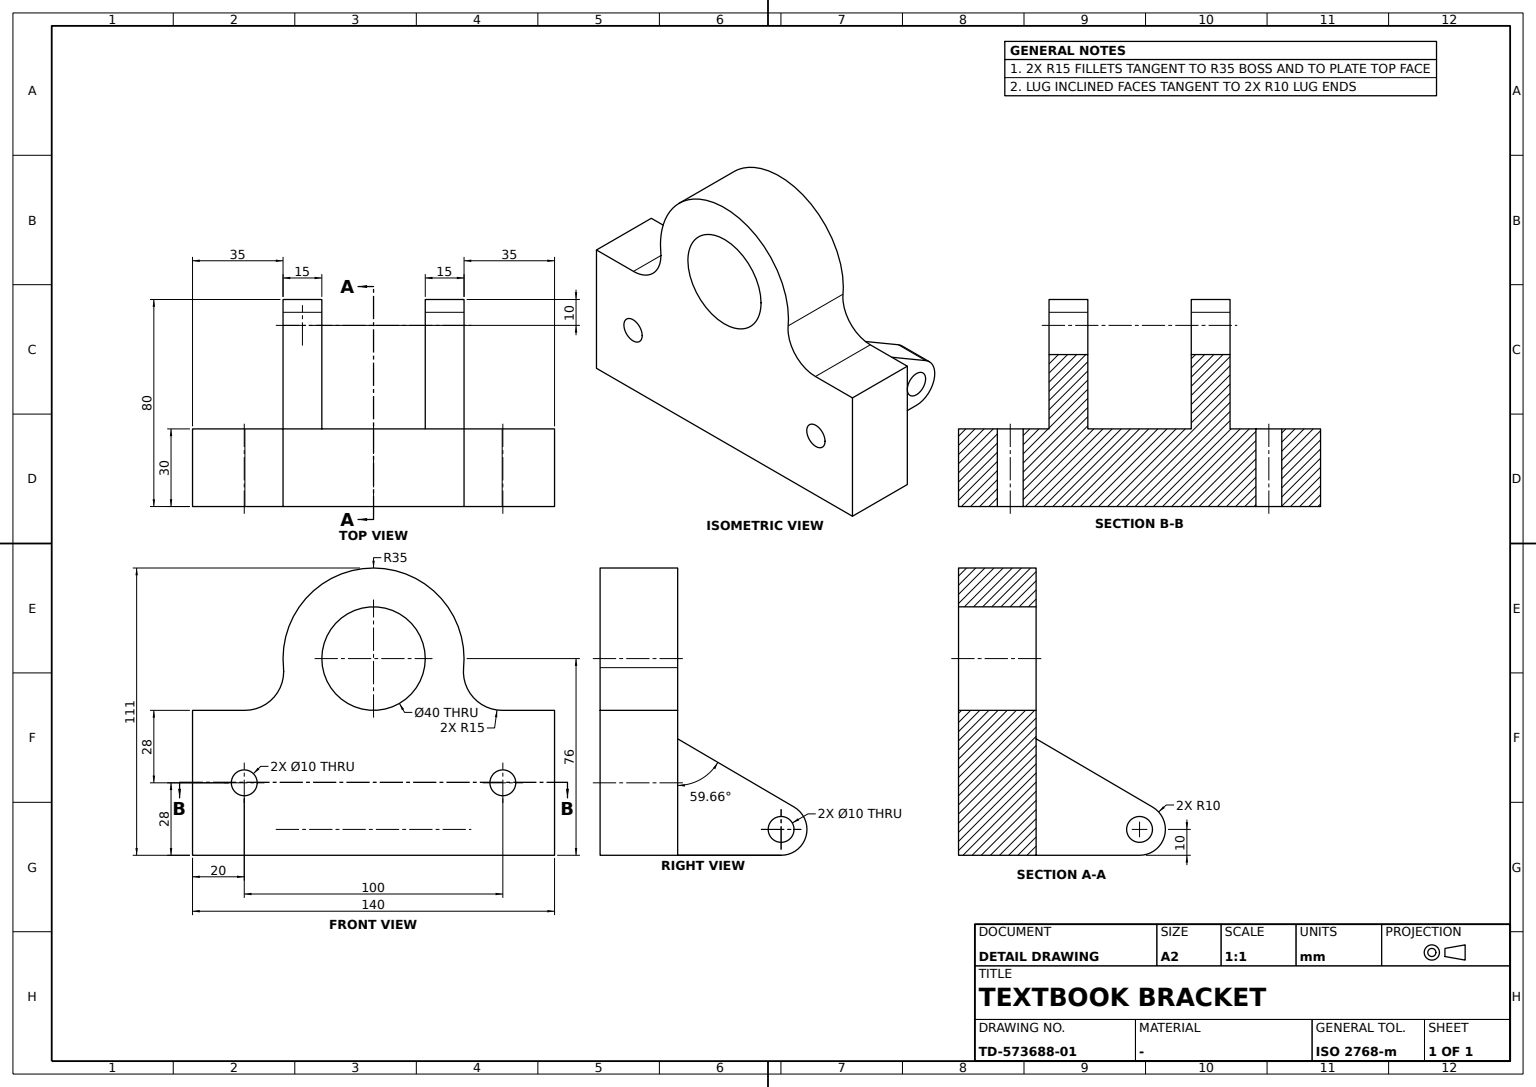
ISO-10303-21;
HEADER;
FILE_DESCRIPTION((''),'2;1');
FILE_NAME('','',(''),(''),'','','');
FILE_SCHEMA(('AUTOMOTIVE_DESIGN'));
ENDSEC;
DATA;
#1=APPLICATION_CONTEXT('');
#2=PRODUCT_CONTEXT('',#1,'mechanical');
#3=PRODUCT('','','',(#2));
#4=PRODUCT_DEFINITION_FORMATION('','',#3);
#5=PRODUCT_DEFINITION_CONTEXT('',#1,'design');
#6=PRODUCT_DEFINITION('','',#4,#5);
#7=PRODUCT_DEFINITION_SHAPE('','',#6);
#8=(LENGTH_UNIT()NAMED_UNIT(*)SI_UNIT(.MILLI.,.METRE.));
#9=(NAMED_UNIT(*)PLANE_ANGLE_UNIT()SI_UNIT($,.RADIAN.));
#10=(NAMED_UNIT(*)SI_UNIT($,.STERADIAN.)SOLID_ANGLE_UNIT());
#11=UNCERTAINTY_MEASURE_WITH_UNIT(LENGTH_MEASURE(1.E-05),#8,'distance_accuracy_value','');
#12=(GEOMETRIC_REPRESENTATION_CONTEXT(3)GLOBAL_UNCERTAINTY_ASSIGNED_CONTEXT((#11))GLOBAL_UNIT_ASSIGNED_CONTEXT((#8,#9,#10))REPRESENTATION_CONTEXT('',''));
#13=CARTESIAN_POINT('',(-40.,-20.,0.));
#14=VERTEX_POINT('',#13);
#15=CARTESIAN_POINT('',(-50.,-20.,10.));
#16=VERTEX_POINT('',#15);
#17=CARTESIAN_POINT('',(-40.,-20.,10.));
#18=DIRECTION('',(0.,1.,0.));
#19=DIRECTION('',(-1.,0.,0.));
#20=AXIS2_PLACEMENT_3D('',#17,#18,#19);
#21=CIRCLE('',#20,10.);
#22=EDGE_CURVE('',#14,#16,#21,.T.);
#23=ORIENTED_EDGE('',*,*,#22,.T.);
#24=CARTESIAN_POINT('',(-45.051517,-20.,18.630305));
#25=VERTEX_POINT('',#24);
#26=EDGE_CURVE('',#16,#25,#21,.T.);
#27=ORIENTED_EDGE('',*,*,#26,.T.);
#28=CARTESIAN_POINT('',(0.,-20.,45.));
#29=VERTEX_POINT('',#28);
#30=CARTESIAN_POINT('',(-22.525759,-20.,31.815153));
#31=DIRECTION('',(0.863030549,0.,0.505151731));
#32=VECTOR('',#31,1000.);
#33=LINE('',#30,#32);
#34=EDGE_CURVE('',#25,#29,#33,.T.);
#35=ORIENTED_EDGE('',*,*,#34,.T.);
#36=CARTESIAN_POINT('',(0.,-20.,0.));
#37=VERTEX_POINT('',#36);
#38=CARTESIAN_POINT('',(0.,-20.,22.5));
#39=DIRECTION('',(0.,0.,-1.));
#40=VECTOR('',#39,1000.);
#41=LINE('',#38,#40);
#42=EDGE_CURVE('',#29,#37,#41,.T.);
#43=ORIENTED_EDGE('',*,*,#42,.T.);
#44=CARTESIAN_POINT('',(-20.,-20.,0.));
#45=VECTOR('',#19,1000.);
#46=LINE('',#44,#45);
#47=EDGE_CURVE('',#37,#14,#46,.T.);
#48=ORIENTED_EDGE('',*,*,#47,.T.);
#49=EDGE_LOOP('',(#23,#27,#35,#43,#48));
#50=FACE_OUTER_BOUND('',#49,.T.);
#51=CARTESIAN_POINT('',(-35.,-20.,10.));
#52=VERTEX_POINT('',#51);
#53=CARTESIAN_POINT('',(-45.,-20.,10.));
#54=VERTEX_POINT('',#53);
#55=CIRCLE('',#20,5.);
#56=EDGE_CURVE('',#52,#54,#55,.T.);
#57=ORIENTED_EDGE('',*,*,#56,.F.);
#58=EDGE_CURVE('',#54,#52,#55,.T.);
#59=ORIENTED_EDGE('',*,*,#58,.F.);
#60=EDGE_LOOP('',(#57,#59));
#61=FACE_BOUND('',#60,.T.);
#62=AXIS2_PLACEMENT_3D('',#36,#18,#19);
#63=PLANE('',#62);
#64=ADVANCED_FACE('',(#50,#61),#63,.T.);
#65=ORIENTED_EDGE('',*,*,#22,.F.);
#66=CARTESIAN_POINT('',(-40.,-35.,0.));
#67=VERTEX_POINT('',#66);
#68=CARTESIAN_POINT('',(-40.,-27.5,0.));
#69=DIRECTION('',(0.,-1.,0.));
#70=VECTOR('',#69,1000.);
#71=LINE('',#68,#70);
#72=EDGE_CURVE('',#14,#67,#71,.T.);
#73=ORIENTED_EDGE('',*,*,#72,.T.);
#74=CARTESIAN_POINT('',(-50.,-35.,10.));
#75=VERTEX_POINT('',#74);
#76=CARTESIAN_POINT('',(-40.,-35.,10.));
#77=AXIS2_PLACEMENT_3D('',#76,#18,#19);
#78=CIRCLE('',#77,10.);
#79=EDGE_CURVE('',#67,#75,#78,.T.);
#80=ORIENTED_EDGE('',*,*,#79,.T.);
#81=CARTESIAN_POINT('',(-50.,27.5,10.));
#82=LINE('',#81,#70);
#83=EDGE_CURVE('',#16,#75,#82,.T.);
#84=ORIENTED_EDGE('',*,*,#83,.F.);
#85=EDGE_LOOP('',(#65,#73,#80,#84));
#86=FACE_OUTER_BOUND('',#85,.T.);
#87=CARTESIAN_POINT('',(-40.,27.5,10.));
#88=AXIS2_PLACEMENT_3D('',#87,#69,#19);
#89=CYLINDRICAL_SURFACE('',#88,10.);
#90=ADVANCED_FACE('',(#86),#89,.T.);
#91=CARTESIAN_POINT('',(0.,-34.82456,72.5));
#92=VERTEX_POINT('',#91);
#93=CARTESIAN_POINT('',(30.,-34.82456,72.5));
#94=VERTEX_POINT('',#93);
#95=CARTESIAN_POINT('',(15.,-34.82456,72.5));
#96=DIRECTION('',(1.,0.,0.));
#97=VECTOR('',#96,1000.);
#98=LINE('',#95,#97);
#99=EDGE_CURVE('',#92,#94,#98,.T.);
#100=ORIENTED_EDGE('',*,*,#99,.F.);
#101=CARTESIAN_POINT('',(0.,-34.749372,71.));
#102=VERTEX_POINT('',#101);
#103=CARTESIAN_POINT('',(0.,-49.749372,71.));
#104=AXIS2_PLACEMENT_3D('',#103,#19,#18);
#105=CIRCLE('',#104,15.);
#106=EDGE_CURVE('',#92,#102,#105,.T.);
#107=ORIENTED_EDGE('',*,*,#106,.T.);
#108=CARTESIAN_POINT('',(30.,-34.749372,71.));
#109=VERTEX_POINT('',#108);
#110=CARTESIAN_POINT('',(15.,-34.749372,71.));
#111=LINE('',#110,#45);
#112=EDGE_CURVE('',#109,#102,#111,.T.);
#113=ORIENTED_EDGE('',*,*,#112,.F.);
#114=CARTESIAN_POINT('',(30.,-49.749372,71.));
#115=AXIS2_PLACEMENT_3D('',#114,#19,#18);
#116=CIRCLE('',#115,15.);
#117=EDGE_CURVE('',#94,#109,#116,.T.);
#118=ORIENTED_EDGE('',*,*,#117,.F.);
#119=EDGE_LOOP('',(#100,#107,#113,#118));
#120=FACE_OUTER_BOUND('',#119,.T.);
#121=CARTESIAN_POINT('',(15.,-49.749372,71.));
#122=AXIS2_PLACEMENT_3D('',#121,#19,#18);
#123=CYLINDRICAL_SURFACE('',#122,15.);
#124=ADVANCED_FACE('',(#120),#123,.F.);
#125=CARTESIAN_POINT('',(30.,35.,76.));
#126=VERTEX_POINT('',#125);
#127=CARTESIAN_POINT('',(0.,35.,76.));
#128=VERTEX_POINT('',#127);
#129=CARTESIAN_POINT('',(15.,35.,76.));
#130=LINE('',#129,#45);
#131=EDGE_CURVE('',#126,#128,#130,.T.);
#132=ORIENTED_EDGE('',*,*,#131,.T.);
#133=CARTESIAN_POINT('',(0.,-35.,76.));
#134=VERTEX_POINT('',#133);
#135=CARTESIAN_POINT('',(0.,0.,76.));
#136=AXIS2_PLACEMENT_3D('',#135,#96,#18);
#137=CIRCLE('',#136,35.);
#138=EDGE_CURVE('',#128,#134,#137,.T.);
#139=ORIENTED_EDGE('',*,*,#138,.T.);
#140=CARTESIAN_POINT('',(30.,-35.,76.));
#141=VERTEX_POINT('',#140);
#142=CARTESIAN_POINT('',(15.,-35.,76.));
#143=LINE('',#142,#45);
#144=EDGE_CURVE('',#141,#134,#143,.T.);
#145=ORIENTED_EDGE('',*,*,#144,.F.);
#146=CARTESIAN_POINT('',(30.,0.,76.));
#147=AXIS2_PLACEMENT_3D('',#146,#96,#18);
#148=CIRCLE('',#147,35.);
#149=EDGE_CURVE('',#126,#141,#148,.T.);
#150=ORIENTED_EDGE('',*,*,#149,.F.);
#151=EDGE_LOOP('',(#132,#139,#145,#150));
#152=FACE_OUTER_BOUND('',#151,.T.);
#153=CARTESIAN_POINT('',(15.,0.,76.));
#154=AXIS2_PLACEMENT_3D('',#153,#19,#18);
#155=CYLINDRICAL_SURFACE('',#154,35.);
#156=ADVANCED_FACE('',(#152),#155,.T.);
#157=CARTESIAN_POINT('',(-40.,20.,0.));
#158=VERTEX_POINT('',#157);
#159=CARTESIAN_POINT('',(-40.,35.,0.));
#160=VERTEX_POINT('',#159);
#161=CARTESIAN_POINT('',(-40.,27.5,0.));
#162=VECTOR('',#18,1000.);
#163=LINE('',#161,#162);
#164=EDGE_CURVE('',#158,#160,#163,.T.);
#165=ORIENTED_EDGE('',*,*,#164,.F.);
#166=CARTESIAN_POINT('',(-50.,20.,10.));
#167=VERTEX_POINT('',#166);
#168=CARTESIAN_POINT('',(-40.,20.,10.));
#169=AXIS2_PLACEMENT_3D('',#168,#18,#19);
#170=CIRCLE('',#169,10.);
#171=EDGE_CURVE('',#158,#167,#170,.T.);
#172=ORIENTED_EDGE('',*,*,#171,.T.);
#173=CARTESIAN_POINT('',(-50.,35.,10.));
#174=VERTEX_POINT('',#173);
#175=EDGE_CURVE('',#174,#167,#82,.T.);
#176=ORIENTED_EDGE('',*,*,#175,.F.);
#177=CARTESIAN_POINT('',(-40.,35.,10.));
#178=AXIS2_PLACEMENT_3D('',#177,#18,#19);
#179=CIRCLE('',#178,10.);
#180=EDGE_CURVE('',#160,#174,#179,.T.);
#181=ORIENTED_EDGE('',*,*,#180,.F.);
#182=EDGE_LOOP('',(#165,#172,#176,#181));
#183=FACE_OUTER_BOUND('',#182,.T.);
#184=ADVANCED_FACE('',(#183),#89,.T.);
#185=CARTESIAN_POINT('',(30.,-45.,28.));
#186=VERTEX_POINT('',#185);
#187=CARTESIAN_POINT('',(0.,-45.,28.));
#188=VERTEX_POINT('',#187);
#189=CARTESIAN_POINT('',(15.,-45.,28.));
#190=LINE('',#189,#45);
#191=EDGE_CURVE('',#186,#188,#190,.T.);
#192=ORIENTED_EDGE('',*,*,#191,.T.);
#193=CARTESIAN_POINT('',(0.,-55.,28.));
#194=VERTEX_POINT('',#193);
#195=CARTESIAN_POINT('',(0.,-50.,28.));
#196=AXIS2_PLACEMENT_3D('',#195,#96,#18);
#197=CIRCLE('',#196,5.);
#198=EDGE_CURVE('',#194,#188,#197,.T.);
#199=ORIENTED_EDGE('',*,*,#198,.F.);
#200=CARTESIAN_POINT('',(30.,-55.,28.));
#201=VERTEX_POINT('',#200);
#202=CARTESIAN_POINT('',(15.,-55.,28.));
#203=LINE('',#202,#45);
#204=EDGE_CURVE('',#201,#194,#203,.T.);
#205=ORIENTED_EDGE('',*,*,#204,.F.);
#206=CARTESIAN_POINT('',(30.,-50.,28.));
#207=AXIS2_PLACEMENT_3D('',#206,#96,#18);
#208=CIRCLE('',#207,5.);
#209=EDGE_CURVE('',#201,#186,#208,.T.);
#210=ORIENTED_EDGE('',*,*,#209,.T.);
#211=EDGE_LOOP('',(#192,#199,#205,#210));
#212=FACE_OUTER_BOUND('',#211,.T.);
#213=CARTESIAN_POINT('',(15.,-50.,28.));
#214=AXIS2_PLACEMENT_3D('',#213,#19,#18);
#215=CYLINDRICAL_SURFACE('',#214,5.);
#216=ADVANCED_FACE('',(#212),#215,.F.);
#217=CARTESIAN_POINT('',(0.,70.,56.));
#218=VERTEX_POINT('',#217);
#219=CARTESIAN_POINT('',(0.,49.749372,56.));
#220=VERTEX_POINT('',#219);
#221=CARTESIAN_POINT('',(0.,59.874686,56.));
#222=LINE('',#221,#70);
#223=EDGE_CURVE('',#218,#220,#222,.T.);
#224=ORIENTED_EDGE('',*,*,#223,.T.);
#225=CARTESIAN_POINT('',(30.,49.749372,56.));
#226=VERTEX_POINT('',#225);
#227=CARTESIAN_POINT('',(15.,49.749372,56.));
#228=LINE('',#227,#97);
#229=EDGE_CURVE('',#220,#226,#228,.T.);
#230=ORIENTED_EDGE('',*,*,#229,.T.);
#231=CARTESIAN_POINT('',(30.,70.,56.));
#232=VERTEX_POINT('',#231);
#233=CARTESIAN_POINT('',(30.,59.874686,56.));
#234=LINE('',#233,#70);
#235=EDGE_CURVE('',#232,#226,#234,.T.);
#236=ORIENTED_EDGE('',*,*,#235,.F.);
#237=CARTESIAN_POINT('',(15.,70.,56.));
#238=LINE('',#237,#97);
#239=EDGE_CURVE('',#218,#232,#238,.T.);
#240=ORIENTED_EDGE('',*,*,#239,.F.);
#241=EDGE_LOOP('',(#224,#230,#236,#240));
#242=FACE_OUTER_BOUND('',#241,.T.);
#243=DIRECTION('',(0.,0.,1.));
#244=AXIS2_PLACEMENT_3D('',#217,#243,#69);
#245=PLANE('',#244);
#246=ADVANCED_FACE('',(#242),#245,.T.);
#247=ORIENTED_EDGE('',*,*,#56,.T.);
#248=CARTESIAN_POINT('',(-45.,-35.,10.));
#249=VERTEX_POINT('',#248);
#250=CARTESIAN_POINT('',(-45.,-18.16,10.));
#251=LINE('',#250,#70);
#252=EDGE_CURVE('',#54,#249,#251,.T.);
#253=ORIENTED_EDGE('',*,*,#252,.T.);
#254=CARTESIAN_POINT('',(-35.,-35.,10.));
#255=VERTEX_POINT('',#254);
#256=CIRCLE('',#77,5.);
#257=EDGE_CURVE('',#255,#249,#256,.T.);
#258=ORIENTED_EDGE('',*,*,#257,.F.);
#259=CARTESIAN_POINT('',(-35.,-18.16,10.));
#260=LINE('',#259,#70);
#261=EDGE_CURVE('',#52,#255,#260,.T.);
#262=ORIENTED_EDGE('',*,*,#261,.F.);
#263=EDGE_LOOP('',(#247,#253,#258,#262));
#264=FACE_OUTER_BOUND('',#263,.T.);
#265=CARTESIAN_POINT('',(-40.,-18.16,10.));
#266=AXIS2_PLACEMENT_3D('',#265,#69,#19);
#267=CYLINDRICAL_SURFACE('',#266,5.);
#268=ADVANCED_FACE('',(#264),#267,.F.);
#269=CARTESIAN_POINT('',(0.,-70.,56.));
#270=VERTEX_POINT('',#269);
#271=CARTESIAN_POINT('',(30.,-70.,56.));
#272=VERTEX_POINT('',#271);
#273=CARTESIAN_POINT('',(15.,-70.,56.));
#274=LINE('',#273,#97);
#275=EDGE_CURVE('',#270,#272,#274,.T.);
#276=ORIENTED_EDGE('',*,*,#275,.F.);
#277=CARTESIAN_POINT('',(0.,-70.,0.));
#278=VERTEX_POINT('',#277);
#279=CARTESIAN_POINT('',(0.,-70.,28.));
#280=LINE('',#279,#40);
#281=EDGE_CURVE('',#270,#278,#280,.T.);
#282=ORIENTED_EDGE('',*,*,#281,.T.);
#283=CARTESIAN_POINT('',(30.,-70.,0.));
#284=VERTEX_POINT('',#283);
#285=CARTESIAN_POINT('',(15.,-70.,0.));
#286=LINE('',#285,#97);
#287=EDGE_CURVE('',#278,#284,#286,.T.);
#288=ORIENTED_EDGE('',*,*,#287,.T.);
#289=CARTESIAN_POINT('',(30.,-70.,28.));
#290=LINE('',#289,#40);
#291=EDGE_CURVE('',#272,#284,#290,.T.);
#292=ORIENTED_EDGE('',*,*,#291,.F.);
#293=EDGE_LOOP('',(#276,#282,#288,#292));
#294=FACE_OUTER_BOUND('',#293,.T.);
#295=AXIS2_PLACEMENT_3D('',#277,#18,#243);
#296=PLANE('',#295);
#297=ADVANCED_FACE('',(#294),#296,.F.);
#298=CARTESIAN_POINT('',(-45.051517,20.,18.630305));
#299=VERTEX_POINT('',#298);
#300=EDGE_CURVE('',#167,#299,#170,.T.);
#301=ORIENTED_EDGE('',*,*,#300,.F.);
#302=ORIENTED_EDGE('',*,*,#171,.F.);
#303=CARTESIAN_POINT('',(0.,20.,0.));
#304=VERTEX_POINT('',#303);
#305=CARTESIAN_POINT('',(-20.,20.,0.));
#306=LINE('',#305,#45);
#307=EDGE_CURVE('',#304,#158,#306,.T.);
#308=ORIENTED_EDGE('',*,*,#307,.F.);
#309=CARTESIAN_POINT('',(0.,20.,45.));
#310=VERTEX_POINT('',#309);
#311=CARTESIAN_POINT('',(0.,20.,22.5));
#312=LINE('',#311,#40);
#313=EDGE_CURVE('',#310,#304,#312,.T.);
#314=ORIENTED_EDGE('',*,*,#313,.F.);
#315=CARTESIAN_POINT('',(-22.525759,20.,31.815153));
#316=LINE('',#315,#32);
#317=EDGE_CURVE('',#299,#310,#316,.T.);
#318=ORIENTED_EDGE('',*,*,#317,.F.);
#319=EDGE_LOOP('',(#301,#302,#308,#314,#318));
#320=FACE_OUTER_BOUND('',#319,.T.);
#321=CARTESIAN_POINT('',(-45.,20.,10.));
#322=VERTEX_POINT('',#321);
#323=CARTESIAN_POINT('',(-35.,20.,10.));
#324=VERTEX_POINT('',#323);
#325=CIRCLE('',#169,5.);
#326=EDGE_CURVE('',#322,#324,#325,.T.);
#327=ORIENTED_EDGE('',*,*,#326,.T.);
#328=EDGE_CURVE('',#324,#322,#325,.T.);
#329=ORIENTED_EDGE('',*,*,#328,.T.);
#330=EDGE_LOOP('',(#327,#329));
#331=FACE_BOUND('',#330,.T.);
#332=AXIS2_PLACEMENT_3D('',#303,#18,#19);
#333=PLANE('',#332);
#334=ADVANCED_FACE('',(#320,#331),#333,.F.);
#335=ORIENTED_EDGE('',*,*,#326,.F.);
#336=CARTESIAN_POINT('',(-45.,35.,10.));
#337=VERTEX_POINT('',#336);
#338=EDGE_CURVE('',#337,#322,#251,.T.);
#339=ORIENTED_EDGE('',*,*,#338,.F.);
#340=CARTESIAN_POINT('',(-35.,35.,10.));
#341=VERTEX_POINT('',#340);
#342=CIRCLE('',#178,5.);
#343=EDGE_CURVE('',#337,#341,#342,.T.);
#344=ORIENTED_EDGE('',*,*,#343,.T.);
#345=EDGE_CURVE('',#341,#324,#260,.T.);
#346=ORIENTED_EDGE('',*,*,#345,.T.);
#347=EDGE_LOOP('',(#335,#339,#344,#346));
#348=FACE_OUTER_BOUND('',#347,.T.);
#349=ADVANCED_FACE('',(#348),#267,.F.);
#350=EDGE_CURVE('',#249,#255,#256,.T.);
#351=ORIENTED_EDGE('',*,*,#350,.F.);
#352=ORIENTED_EDGE('',*,*,#252,.F.);
#353=ORIENTED_EDGE('',*,*,#58,.T.);
#354=ORIENTED_EDGE('',*,*,#261,.T.);
#355=EDGE_LOOP('',(#351,#352,#353,#354));
#356=FACE_OUTER_BOUND('',#355,.T.);
#357=ADVANCED_FACE('',(#356),#267,.F.);
#358=CARTESIAN_POINT('',(0.,70.,0.));
#359=VERTEX_POINT('',#358);
#360=CARTESIAN_POINT('',(30.,70.,0.));
#361=VERTEX_POINT('',#360);
#362=CARTESIAN_POINT('',(15.,70.,0.));
#363=LINE('',#362,#97);
#364=EDGE_CURVE('',#359,#361,#363,.T.);
#365=ORIENTED_EDGE('',*,*,#364,.T.);
#366=CARTESIAN_POINT('',(30.,0.,0.));
#367=LINE('',#366,#162);
#368=EDGE_CURVE('',#284,#361,#367,.T.);
#369=ORIENTED_EDGE('',*,*,#368,.F.);
#370=ORIENTED_EDGE('',*,*,#287,.F.);
#371=CARTESIAN_POINT('',(0.,-35.,0.));
#372=VERTEX_POINT('',#371);
#373=CARTESIAN_POINT('',(0.,-52.5,0.));
#374=LINE('',#373,#162);
#375=EDGE_CURVE('',#278,#372,#374,.T.);
#376=ORIENTED_EDGE('',*,*,#375,.T.);
#377=CARTESIAN_POINT('',(-20.,-35.,0.));
#378=LINE('',#377,#45);
#379=EDGE_CURVE('',#372,#67,#378,.T.);
#380=ORIENTED_EDGE('',*,*,#379,.T.);
#381=ORIENTED_EDGE('',*,*,#72,.F.);
#382=ORIENTED_EDGE('',*,*,#47,.F.);
#383=CARTESIAN_POINT('',(0.,0.,0.));
#384=LINE('',#383,#162);
#385=EDGE_CURVE('',#37,#304,#384,.T.);
#386=ORIENTED_EDGE('',*,*,#385,.T.);
#387=ORIENTED_EDGE('',*,*,#307,.T.);
#388=ORIENTED_EDGE('',*,*,#164,.T.);
#389=CARTESIAN_POINT('',(0.,35.,0.));
#390=VERTEX_POINT('',#389);
#391=CARTESIAN_POINT('',(-20.,35.,0.));
#392=LINE('',#391,#45);
#393=EDGE_CURVE('',#390,#160,#392,.T.);
#394=ORIENTED_EDGE('',*,*,#393,.F.);
#395=CARTESIAN_POINT('',(0.,52.5,0.));
#396=LINE('',#395,#162);
#397=EDGE_CURVE('',#390,#359,#396,.T.);
#398=ORIENTED_EDGE('',*,*,#397,.T.);
#399=EDGE_LOOP('',(#365,#369,#370,#376,#380,#381,#382,#386,#387,#388,#394,#398));
#400=FACE_OUTER_BOUND('',#399,.T.);
#401=AXIS2_PLACEMENT_3D('',#277,#39,#18);
#402=PLANE('',#401);
#403=ADVANCED_FACE('',(#400),#402,.T.);
#404=ORIENTED_EDGE('',*,*,#83,.T.);
#405=CARTESIAN_POINT('',(-45.051517,-35.,18.630305));
#406=VERTEX_POINT('',#405);
#407=EDGE_CURVE('',#75,#406,#78,.T.);
#408=ORIENTED_EDGE('',*,*,#407,.T.);
#409=CARTESIAN_POINT('',(-45.051517,27.5,18.630305));
#410=LINE('',#409,#70);
#411=EDGE_CURVE('',#25,#406,#410,.T.);
#412=ORIENTED_EDGE('',*,*,#411,.F.);
#413=ORIENTED_EDGE('',*,*,#26,.F.);
#414=EDGE_LOOP('',(#404,#408,#412,#413));
#415=FACE_OUTER_BOUND('',#414,.T.);
#416=ADVANCED_FACE('',(#415),#89,.T.);
#417=CARTESIAN_POINT('',(0.,34.82456,72.5));
#418=VERTEX_POINT('',#417);
#419=CARTESIAN_POINT('',(30.,34.82456,72.5));
#420=VERTEX_POINT('',#419);
#421=CARTESIAN_POINT('',(15.,34.82456,72.5));
#422=LINE('',#421,#97);
#423=EDGE_CURVE('',#418,#420,#422,.T.);
#424=ORIENTED_EDGE('',*,*,#423,.F.);
#425=EDGE_CURVE('',#418,#128,#137,.T.);
#426=ORIENTED_EDGE('',*,*,#425,.T.);
#427=ORIENTED_EDGE('',*,*,#131,.F.);
#428=EDGE_CURVE('',#420,#126,#148,.T.);
#429=ORIENTED_EDGE('',*,*,#428,.F.);
#430=EDGE_LOOP('',(#424,#426,#427,#429));
#431=FACE_OUTER_BOUND('',#430,.T.);
#432=ADVANCED_FACE('',(#431),#155,.T.);
#433=ORIENTED_EDGE('',*,*,#343,.F.);
#434=EDGE_CURVE('',#341,#337,#342,.T.);
#435=ORIENTED_EDGE('',*,*,#434,.F.);
#436=EDGE_LOOP('',(#433,#435));
#437=FACE_BOUND('',#436,.T.);
#438=ORIENTED_EDGE('',*,*,#393,.T.);
#439=ORIENTED_EDGE('',*,*,#180,.T.);
#440=CARTESIAN_POINT('',(-45.051517,35.,18.630305));
#441=VERTEX_POINT('',#440);
#442=EDGE_CURVE('',#174,#441,#179,.T.);
#443=ORIENTED_EDGE('',*,*,#442,.T.);
#444=CARTESIAN_POINT('',(0.,35.,45.));
#445=VERTEX_POINT('',#444);
#446=CARTESIAN_POINT('',(-22.525759,35.,31.815153));
#447=LINE('',#446,#32);
#448=EDGE_CURVE('',#441,#445,#447,.T.);
#449=ORIENTED_EDGE('',*,*,#448,.T.);
#450=CARTESIAN_POINT('',(0.,35.,22.5));
#451=LINE('',#450,#40);
#452=EDGE_CURVE('',#445,#390,#451,.T.);
#453=ORIENTED_EDGE('',*,*,#452,.T.);
#454=EDGE_LOOP('',(#438,#439,#443,#449,#453));
#455=FACE_OUTER_BOUND('',#454,.T.);
#456=AXIS2_PLACEMENT_3D('',#389,#18,#19);
#457=PLANE('',#456);
#458=ADVANCED_FACE('',(#437,#455),#457,.T.);
#459=ORIENTED_EDGE('',*,*,#350,.T.);
#460=ORIENTED_EDGE('',*,*,#257,.T.);
#461=EDGE_LOOP('',(#459,#460));
#462=FACE_BOUND('',#461,.T.);
#463=ORIENTED_EDGE('',*,*,#407,.F.);
#464=ORIENTED_EDGE('',*,*,#79,.F.);
#465=ORIENTED_EDGE('',*,*,#379,.F.);
#466=CARTESIAN_POINT('',(0.,-35.,45.));
#467=VERTEX_POINT('',#466);
#468=CARTESIAN_POINT('',(0.,-35.,22.5));
#469=LINE('',#468,#40);
#470=EDGE_CURVE('',#467,#372,#469,.T.);
#471=ORIENTED_EDGE('',*,*,#470,.F.);
#472=CARTESIAN_POINT('',(-22.525759,-35.,31.815153));
#473=LINE('',#472,#32);
#474=EDGE_CURVE('',#406,#467,#473,.T.);
#475=ORIENTED_EDGE('',*,*,#474,.F.);
#476=EDGE_LOOP('',(#463,#464,#465,#471,#475));
#477=FACE_OUTER_BOUND('',#476,.T.);
#478=AXIS2_PLACEMENT_3D('',#371,#18,#19);
#479=PLANE('',#478);
#480=ADVANCED_FACE('',(#462,#477),#479,.F.);
#481=ORIENTED_EDGE('',*,*,#198,.T.);
#482=EDGE_CURVE('',#188,#194,#197,.T.);
#483=ORIENTED_EDGE('',*,*,#482,.T.);
#484=EDGE_LOOP('',(#481,#483));
#485=FACE_BOUND('',#484,.T.);
#486=ORIENTED_EDGE('',*,*,#223,.F.);
#487=CARTESIAN_POINT('',(0.,70.,28.));
#488=VECTOR('',#243,1000.);
#489=LINE('',#487,#488);
#490=EDGE_CURVE('',#359,#218,#489,.T.);
#491=ORIENTED_EDGE('',*,*,#490,.F.);
#492=ORIENTED_EDGE('',*,*,#397,.F.);
#493=ORIENTED_EDGE('',*,*,#452,.F.);
#494=CARTESIAN_POINT('',(0.,27.5,45.));
#495=LINE('',#494,#162);
#496=EDGE_CURVE('',#310,#445,#495,.T.);
#497=ORIENTED_EDGE('',*,*,#496,.F.);
#498=ORIENTED_EDGE('',*,*,#313,.T.);
#499=ORIENTED_EDGE('',*,*,#385,.F.);
#500=ORIENTED_EDGE('',*,*,#42,.F.);
#501=CARTESIAN_POINT('',(0.,-27.5,45.));
#502=LINE('',#501,#70);
#503=EDGE_CURVE('',#29,#467,#502,.T.);
#504=ORIENTED_EDGE('',*,*,#503,.T.);
#505=ORIENTED_EDGE('',*,*,#470,.T.);
#506=ORIENTED_EDGE('',*,*,#375,.F.);
#507=ORIENTED_EDGE('',*,*,#281,.F.);
#508=CARTESIAN_POINT('',(0.,-49.749372,56.));
#509=VERTEX_POINT('',#508);
#510=CARTESIAN_POINT('',(0.,-59.874686,56.));
#511=LINE('',#510,#70);
#512=EDGE_CURVE('',#509,#270,#511,.T.);
#513=ORIENTED_EDGE('',*,*,#512,.F.);
#514=EDGE_CURVE('',#102,#509,#105,.T.);
#515=ORIENTED_EDGE('',*,*,#514,.F.);
#516=ORIENTED_EDGE('',*,*,#106,.F.);
#517=EDGE_CURVE('',#134,#92,#137,.T.);
#518=ORIENTED_EDGE('',*,*,#517,.F.);
#519=ORIENTED_EDGE('',*,*,#138,.F.);
#520=ORIENTED_EDGE('',*,*,#425,.F.);
#521=CARTESIAN_POINT('',(0.,49.749372,71.));
#522=AXIS2_PLACEMENT_3D('',#521,#19,#18);
#523=CIRCLE('',#522,15.);
#524=EDGE_CURVE('',#220,#418,#523,.T.);
#525=ORIENTED_EDGE('',*,*,#524,.F.);
#526=EDGE_LOOP('',(#486,#491,#492,#493,#497,#498,#499,#500,#504,#505,#506,#507,#513,#515,#516,#518,#519,#520,#525));
#527=FACE_OUTER_BOUND('',#526,.T.);
#528=CARTESIAN_POINT('',(0.,45.,28.));
#529=VERTEX_POINT('',#528);
#530=CARTESIAN_POINT('',(0.,55.,28.));
#531=VERTEX_POINT('',#530);
#532=CARTESIAN_POINT('',(0.,50.,28.));
#533=AXIS2_PLACEMENT_3D('',#532,#96,#18);
#534=CIRCLE('',#533,5.);
#535=EDGE_CURVE('',#529,#531,#534,.T.);
#536=ORIENTED_EDGE('',*,*,#535,.T.);
#537=EDGE_CURVE('',#531,#529,#534,.T.);
#538=ORIENTED_EDGE('',*,*,#537,.T.);
#539=EDGE_LOOP('',(#536,#538));
#540=FACE_BOUND('',#539,.T.);
#541=CARTESIAN_POINT('',(0.,20.,76.));
#542=VERTEX_POINT('',#541);
#543=CARTESIAN_POINT('',(0.,-20.,76.));
#544=VERTEX_POINT('',#543);
#545=CIRCLE('',#136,20.);
#546=EDGE_CURVE('',#542,#544,#545,.T.);
#547=ORIENTED_EDGE('',*,*,#546,.T.);
#548=EDGE_CURVE('',#544,#542,#545,.T.);
#549=ORIENTED_EDGE('',*,*,#548,.T.);
#550=EDGE_LOOP('',(#547,#549));
#551=FACE_BOUND('',#550,.T.);
#552=AXIS2_PLACEMENT_3D('',#383,#96,#18);
#553=PLANE('',#552);
#554=ADVANCED_FACE('',(#485,#527,#540,#551),#553,.F.);
#555=ORIENTED_EDGE('',*,*,#517,.T.);
#556=ORIENTED_EDGE('',*,*,#99,.T.);
#557=EDGE_CURVE('',#141,#94,#148,.T.);
#558=ORIENTED_EDGE('',*,*,#557,.F.);
#559=ORIENTED_EDGE('',*,*,#144,.T.);
#560=EDGE_LOOP('',(#555,#556,#558,#559));
#561=FACE_OUTER_BOUND('',#560,.T.);
#562=ADVANCED_FACE('',(#561),#155,.T.);
#563=ORIENTED_EDGE('',*,*,#512,.T.);
#564=ORIENTED_EDGE('',*,*,#275,.T.);
#565=CARTESIAN_POINT('',(30.,-49.749372,56.));
#566=VERTEX_POINT('',#565);
#567=CARTESIAN_POINT('',(30.,-59.874686,56.));
#568=LINE('',#567,#70);
#569=EDGE_CURVE('',#566,#272,#568,.T.);
#570=ORIENTED_EDGE('',*,*,#569,.F.);
#571=CARTESIAN_POINT('',(15.,-49.749372,56.));
#572=LINE('',#571,#97);
#573=EDGE_CURVE('',#509,#566,#572,.T.);
#574=ORIENTED_EDGE('',*,*,#573,.F.);
#575=EDGE_LOOP('',(#563,#564,#570,#574));
#576=FACE_OUTER_BOUND('',#575,.T.);
#577=ADVANCED_FACE('',(#576),#245,.T.);
#578=ORIENTED_EDGE('',*,*,#34,.F.);
#579=ORIENTED_EDGE('',*,*,#411,.T.);
#580=ORIENTED_EDGE('',*,*,#474,.T.);
#581=ORIENTED_EDGE('',*,*,#503,.F.);
#582=EDGE_LOOP('',(#578,#579,#580,#581));
#583=FACE_OUTER_BOUND('',#582,.T.);
#584=CARTESIAN_POINT('',(0.,0.,45.));
#585=DIRECTION('',(0.505151731,0.,-0.863030549));
#586=DIRECTION('',(-0.863030549,0.,-0.505151731));
#587=AXIS2_PLACEMENT_3D('',#584,#585,#586);
#588=PLANE('',#587);
#589=ADVANCED_FACE('',(#583),#588,.F.);
#590=ORIENTED_EDGE('',*,*,#537,.F.);
#591=CARTESIAN_POINT('',(30.,55.,28.));
#592=VERTEX_POINT('',#591);
#593=CARTESIAN_POINT('',(15.,55.,28.));
#594=LINE('',#593,#45);
#595=EDGE_CURVE('',#592,#531,#594,.T.);
#596=ORIENTED_EDGE('',*,*,#595,.F.);
#597=CARTESIAN_POINT('',(30.,45.,28.));
#598=VERTEX_POINT('',#597);
#599=CARTESIAN_POINT('',(30.,50.,28.));
#600=AXIS2_PLACEMENT_3D('',#599,#96,#18);
#601=CIRCLE('',#600,5.);
#602=EDGE_CURVE('',#592,#598,#601,.T.);
#603=ORIENTED_EDGE('',*,*,#602,.T.);
#604=CARTESIAN_POINT('',(15.,45.,28.));
#605=LINE('',#604,#45);
#606=EDGE_CURVE('',#598,#529,#605,.T.);
#607=ORIENTED_EDGE('',*,*,#606,.T.);
#608=EDGE_LOOP('',(#590,#596,#603,#607));
#609=FACE_OUTER_BOUND('',#608,.T.);
#610=CARTESIAN_POINT('',(15.,50.,28.));
#611=AXIS2_PLACEMENT_3D('',#610,#19,#18);
#612=CYLINDRICAL_SURFACE('',#611,5.);
#613=ADVANCED_FACE('',(#609),#612,.F.);
#614=ORIENTED_EDGE('',*,*,#112,.T.);
#615=ORIENTED_EDGE('',*,*,#514,.T.);
#616=ORIENTED_EDGE('',*,*,#573,.T.);
#617=EDGE_CURVE('',#109,#566,#116,.T.);
#618=ORIENTED_EDGE('',*,*,#617,.F.);
#619=EDGE_LOOP('',(#614,#615,#616,#618));
#620=FACE_OUTER_BOUND('',#619,.T.);
#621=ADVANCED_FACE('',(#620),#123,.F.);
#622=ORIENTED_EDGE('',*,*,#482,.F.);
#623=ORIENTED_EDGE('',*,*,#191,.F.);
#624=EDGE_CURVE('',#186,#201,#208,.T.);
#625=ORIENTED_EDGE('',*,*,#624,.T.);
#626=ORIENTED_EDGE('',*,*,#204,.T.);
#627=EDGE_LOOP('',(#622,#623,#625,#626));
#628=FACE_OUTER_BOUND('',#627,.T.);
#629=ADVANCED_FACE('',(#628),#215,.F.);
#630=ORIENTED_EDGE('',*,*,#338,.T.);
#631=ORIENTED_EDGE('',*,*,#328,.F.);
#632=ORIENTED_EDGE('',*,*,#345,.F.);
#633=ORIENTED_EDGE('',*,*,#434,.T.);
#634=EDGE_LOOP('',(#630,#631,#632,#633));
#635=FACE_OUTER_BOUND('',#634,.T.);
#636=ADVANCED_FACE('',(#635),#267,.F.);
#637=CARTESIAN_POINT('',(30.,49.749372,71.));
#638=AXIS2_PLACEMENT_3D('',#637,#19,#18);
#639=CIRCLE('',#638,15.);
#640=EDGE_CURVE('',#226,#420,#639,.T.);
#641=ORIENTED_EDGE('',*,*,#640,.T.);
#642=ORIENTED_EDGE('',*,*,#428,.T.);
#643=ORIENTED_EDGE('',*,*,#149,.T.);
#644=ORIENTED_EDGE('',*,*,#557,.T.);
#645=ORIENTED_EDGE('',*,*,#117,.T.);
#646=ORIENTED_EDGE('',*,*,#617,.T.);
#647=ORIENTED_EDGE('',*,*,#569,.T.);
#648=ORIENTED_EDGE('',*,*,#291,.T.);
#649=ORIENTED_EDGE('',*,*,#368,.T.);
#650=CARTESIAN_POINT('',(30.,70.,28.));
#651=LINE('',#650,#488);
#652=EDGE_CURVE('',#361,#232,#651,.T.);
#653=ORIENTED_EDGE('',*,*,#652,.T.);
#654=ORIENTED_EDGE('',*,*,#235,.T.);
#655=EDGE_LOOP('',(#641,#642,#643,#644,#645,#646,#647,#648,#649,#653,#654));
#656=FACE_OUTER_BOUND('',#655,.T.);
#657=ORIENTED_EDGE('',*,*,#209,.F.);
#658=ORIENTED_EDGE('',*,*,#624,.F.);
#659=EDGE_LOOP('',(#657,#658));
#660=FACE_BOUND('',#659,.T.);
#661=EDGE_CURVE('',#598,#592,#601,.T.);
#662=ORIENTED_EDGE('',*,*,#661,.F.);
#663=ORIENTED_EDGE('',*,*,#602,.F.);
#664=EDGE_LOOP('',(#662,#663));
#665=FACE_BOUND('',#664,.T.);
#666=CARTESIAN_POINT('',(30.,-20.,76.));
#667=VERTEX_POINT('',#666);
#668=CARTESIAN_POINT('',(30.,20.,76.));
#669=VERTEX_POINT('',#668);
#670=CIRCLE('',#147,20.);
#671=EDGE_CURVE('',#667,#669,#670,.T.);
#672=ORIENTED_EDGE('',*,*,#671,.F.);
#673=EDGE_CURVE('',#669,#667,#670,.T.);
#674=ORIENTED_EDGE('',*,*,#673,.F.);
#675=EDGE_LOOP('',(#672,#674));
#676=FACE_BOUND('',#675,.T.);
#677=AXIS2_PLACEMENT_3D('',#366,#96,#18);
#678=PLANE('',#677);
#679=ADVANCED_FACE('',(#656,#660,#665,#676),#678,.T.);
#680=LINE('',#409,#162);
#681=EDGE_CURVE('',#299,#441,#680,.T.);
#682=ORIENTED_EDGE('',*,*,#681,.T.);
#683=ORIENTED_EDGE('',*,*,#442,.F.);
#684=ORIENTED_EDGE('',*,*,#175,.T.);
#685=ORIENTED_EDGE('',*,*,#300,.T.);
#686=EDGE_LOOP('',(#682,#683,#684,#685));
#687=FACE_OUTER_BOUND('',#686,.T.);
#688=ADVANCED_FACE('',(#687),#89,.T.);
#689=CARTESIAN_POINT('',(15.,20.,76.));
#690=LINE('',#689,#45);
#691=EDGE_CURVE('',#669,#542,#690,.T.);
#692=ORIENTED_EDGE('',*,*,#691,.T.);
#693=ORIENTED_EDGE('',*,*,#548,.F.);
#694=CARTESIAN_POINT('',(15.,-20.,76.));
#695=LINE('',#694,#45);
#696=EDGE_CURVE('',#667,#544,#695,.T.);
#697=ORIENTED_EDGE('',*,*,#696,.F.);
#698=ORIENTED_EDGE('',*,*,#671,.T.);
#699=EDGE_LOOP('',(#692,#693,#697,#698));
#700=FACE_OUTER_BOUND('',#699,.T.);
#701=CYLINDRICAL_SURFACE('',#154,20.);
#702=ADVANCED_FACE('',(#700),#701,.F.);
#703=ORIENTED_EDGE('',*,*,#691,.F.);
#704=ORIENTED_EDGE('',*,*,#673,.T.);
#705=ORIENTED_EDGE('',*,*,#696,.T.);
#706=ORIENTED_EDGE('',*,*,#546,.F.);
#707=EDGE_LOOP('',(#703,#704,#705,#706));
#708=FACE_OUTER_BOUND('',#707,.T.);
#709=ADVANCED_FACE('',(#708),#701,.F.);
#710=ORIENTED_EDGE('',*,*,#317,.T.);
#711=ORIENTED_EDGE('',*,*,#496,.T.);
#712=ORIENTED_EDGE('',*,*,#448,.F.);
#713=ORIENTED_EDGE('',*,*,#681,.F.);
#714=EDGE_LOOP('',(#710,#711,#712,#713));
#715=FACE_OUTER_BOUND('',#714,.T.);
#716=ADVANCED_FACE('',(#715),#588,.F.);
#717=ORIENTED_EDGE('',*,*,#239,.T.);
#718=ORIENTED_EDGE('',*,*,#652,.F.);
#719=ORIENTED_EDGE('',*,*,#364,.F.);
#720=ORIENTED_EDGE('',*,*,#490,.T.);
#721=EDGE_LOOP('',(#717,#718,#719,#720));
#722=FACE_OUTER_BOUND('',#721,.T.);
#723=AXIS2_PLACEMENT_3D('',#358,#18,#243);
#724=PLANE('',#723);
#725=ADVANCED_FACE('',(#722),#724,.T.);
#726=ORIENTED_EDGE('',*,*,#606,.F.);
#727=ORIENTED_EDGE('',*,*,#661,.T.);
#728=ORIENTED_EDGE('',*,*,#595,.T.);
#729=ORIENTED_EDGE('',*,*,#535,.F.);
#730=EDGE_LOOP('',(#726,#727,#728,#729));
#731=FACE_OUTER_BOUND('',#730,.T.);
#732=ADVANCED_FACE('',(#731),#612,.F.);
#733=ORIENTED_EDGE('',*,*,#524,.T.);
#734=ORIENTED_EDGE('',*,*,#423,.T.);
#735=ORIENTED_EDGE('',*,*,#640,.F.);
#736=ORIENTED_EDGE('',*,*,#229,.F.);
#737=EDGE_LOOP('',(#733,#734,#735,#736));
#738=FACE_OUTER_BOUND('',#737,.T.);
#739=CARTESIAN_POINT('',(15.,49.749372,71.));
#740=AXIS2_PLACEMENT_3D('',#739,#19,#18);
#741=CYLINDRICAL_SURFACE('',#740,15.);
#742=ADVANCED_FACE('',(#738),#741,.F.);
#743=CLOSED_SHELL('',(#64,#90,#124,#156,#184,#216,#246,#268,#297,#334,#349,#357,#403,#416,#432,#458,#480,#554,#562,#577,#589,#613,#621,#629,#636,#679,#688,#702,#709,#716,#725,#732,#742));
#744=MANIFOLD_SOLID_BREP('',#743);
#745=ADVANCED_BREP_SHAPE_REPRESENTATION('',(#744),#12);
#746=SHAPE_DEFINITION_REPRESENTATION(#7,#745);
ENDSEC;
END-ISO-10303-21;
